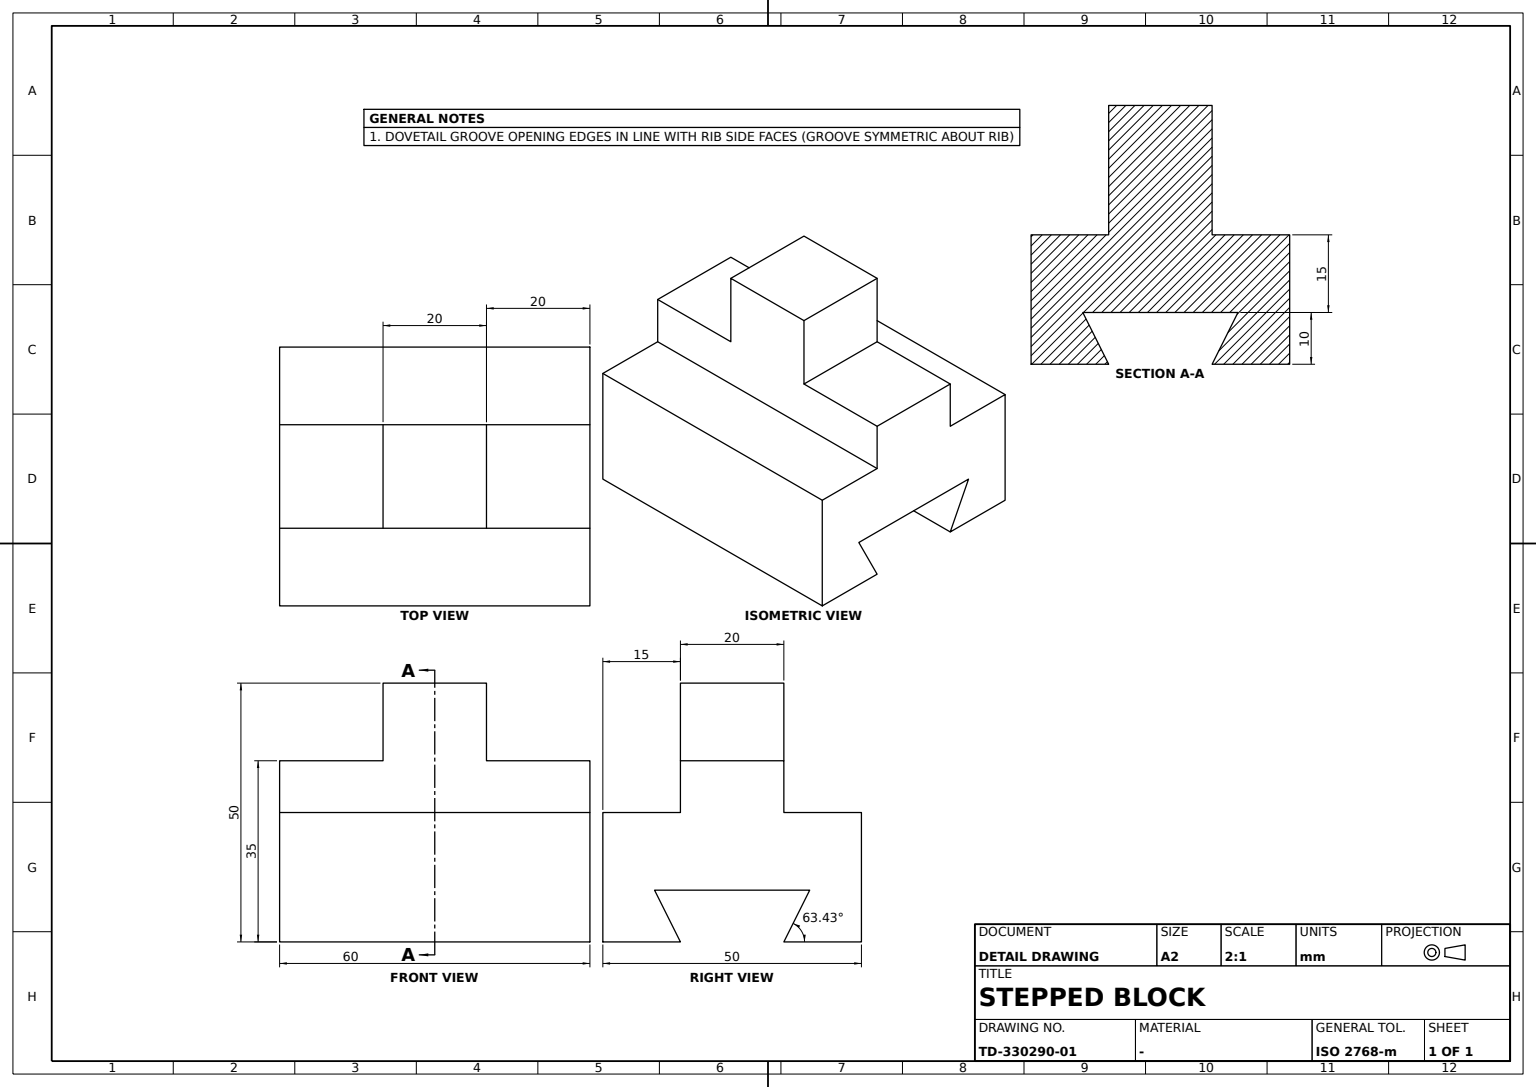
ISO-10303-21;
HEADER;
FILE_DESCRIPTION((''),'2;1');
FILE_NAME('','',(''),(''),'','','');
FILE_SCHEMA(('AUTOMOTIVE_DESIGN'));
ENDSEC;
DATA;
#1=APPLICATION_CONTEXT('');
#2=PRODUCT_CONTEXT('',#1,'mechanical');
#3=PRODUCT('','','',(#2));
#4=PRODUCT_DEFINITION_FORMATION('','',#3);
#5=PRODUCT_DEFINITION_CONTEXT('',#1,'design');
#6=PRODUCT_DEFINITION('','',#4,#5);
#7=PRODUCT_DEFINITION_SHAPE('','',#6);
#8=(LENGTH_UNIT()NAMED_UNIT(*)SI_UNIT(.MILLI.,.METRE.));
#9=(NAMED_UNIT(*)PLANE_ANGLE_UNIT()SI_UNIT($,.RADIAN.));
#10=(NAMED_UNIT(*)SI_UNIT($,.STERADIAN.)SOLID_ANGLE_UNIT());
#11=UNCERTAINTY_MEASURE_WITH_UNIT(LENGTH_MEASURE(0.005),#8,'distance_accuracy_value','');
#12=(GEOMETRIC_REPRESENTATION_CONTEXT(3)GLOBAL_UNCERTAINTY_ASSIGNED_CONTEXT((#11))GLOBAL_UNIT_ASSIGNED_CONTEXT((#8,#9,#10))REPRESENTATION_CONTEXT('',''));
#13=CARTESIAN_POINT('',(30.,-10.,-12.5));
#14=VERTEX_POINT('',#13);
#15=CARTESIAN_POINT('',(-30.,-10.,-12.5));
#16=VERTEX_POINT('',#15);
#17=CARTESIAN_POINT('',(60.,-10.,-12.5));
#18=DIRECTION('',(-1.,0.,0.));
#19=VECTOR('',#18,1000.);
#20=LINE('',#17,#19);
#21=EDGE_CURVE('',#14,#16,#20,.T.);
#22=ORIENTED_EDGE('',*,*,#21,.T.);
#23=CARTESIAN_POINT('',(-30.,-15.,-2.5));
#24=VERTEX_POINT('',#23);
#25=CARTESIAN_POINT('',(-30.,-13.,-6.5));
#26=DIRECTION('',(0.,-0.447213595,0.894427191));
#27=VECTOR('',#26,1000.);
#28=LINE('',#25,#27);
#29=EDGE_CURVE('',#16,#24,#28,.T.);
#30=ORIENTED_EDGE('',*,*,#29,.T.);
#31=CARTESIAN_POINT('',(30.,-15.,-2.5));
#32=VERTEX_POINT('',#31);
#33=CARTESIAN_POINT('',(60.,-15.,-2.5));
#34=LINE('',#33,#19);
#35=EDGE_CURVE('',#24,#32,#34,.F.);
#36=ORIENTED_EDGE('',*,*,#35,.T.);
#37=CARTESIAN_POINT('',(30.,-13.,-6.5));
#38=LINE('',#37,#27);
#39=EDGE_CURVE('',#14,#32,#38,.T.);
#40=ORIENTED_EDGE('',*,*,#39,.F.);
#41=EDGE_LOOP('',(#22,#30,#36,#40));
#42=FACE_BOUND('',#41,.T.);
#43=DIRECTION('',(0.,0.894427191,0.447213595));
#44=AXIS2_PLACEMENT_3D('',#33,#43,#26);
#45=PLANE('',#44);
#46=ADVANCED_FACE('',(#42),#45,.T.);
#47=CARTESIAN_POINT('',(10.,-10.,22.5));
#48=VERTEX_POINT('',#47);
#49=CARTESIAN_POINT('',(10.,-10.,37.5));
#50=VERTEX_POINT('',#49);
#51=DIRECTION('',(0.,0.,1.));
#52=VECTOR('',#51,1000.);
#53=LINE('',#47,#52);
#54=EDGE_CURVE('',#48,#50,#53,.T.);
#55=ORIENTED_EDGE('',*,*,#54,.F.);
#56=CARTESIAN_POINT('',(10.,10.,22.5));
#57=VERTEX_POINT('',#56);
#58=DIRECTION('',(0.,1.,0.));
#59=VECTOR('',#58,1000.);
#60=LINE('',#47,#59);
#61=EDGE_CURVE('',#48,#57,#60,.T.);
#62=ORIENTED_EDGE('',*,*,#61,.T.);
#63=CARTESIAN_POINT('',(10.,10.,37.5));
#64=VERTEX_POINT('',#63);
#65=LINE('',#56,#52);
#66=EDGE_CURVE('',#57,#64,#65,.T.);
#67=ORIENTED_EDGE('',*,*,#66,.T.);
#68=LINE('',#49,#59);
#69=EDGE_CURVE('',#50,#64,#68,.T.);
#70=ORIENTED_EDGE('',*,*,#69,.F.);
#71=EDGE_LOOP('',(#55,#62,#67,#70));
#72=FACE_BOUND('',#71,.T.);
#73=AXIS2_PLACEMENT_3D('',#47,#18,#51);
#74=PLANE('',#73);
#75=ADVANCED_FACE('',(#72),#74,.F.);
#76=CARTESIAN_POINT('',(-30.,-25.,12.5));
#77=VERTEX_POINT('',#76);
#78=CARTESIAN_POINT('',(-30.,-25.,-12.5));
#79=VERTEX_POINT('',#78);
#80=DIRECTION('',(0.,0.,-1.));
#81=VECTOR('',#80,1000.);
#82=LINE('',#76,#81);
#83=EDGE_CURVE('',#77,#79,#82,.T.);
#84=ORIENTED_EDGE('',*,*,#83,.F.);
#85=CARTESIAN_POINT('',(-30.,-10.,12.5));
#86=VERTEX_POINT('',#85);
#87=CARTESIAN_POINT('',(-30.,25.,12.5));
#88=DIRECTION('',(0.,-1.,0.));
#89=VECTOR('',#88,1000.);
#90=LINE('',#87,#89);
#91=EDGE_CURVE('',#86,#77,#90,.T.);
#92=ORIENTED_EDGE('',*,*,#91,.F.);
#93=CARTESIAN_POINT('',(-30.,-10.,22.5));
#94=VERTEX_POINT('',#93);
#95=LINE('',#85,#52);
#96=EDGE_CURVE('',#86,#94,#95,.T.);
#97=ORIENTED_EDGE('',*,*,#96,.T.);
#98=CARTESIAN_POINT('',(-30.,10.,22.5));
#99=VERTEX_POINT('',#98);
#100=LINE('',#93,#59);
#101=EDGE_CURVE('',#94,#99,#100,.T.);
#102=ORIENTED_EDGE('',*,*,#101,.T.);
#103=CARTESIAN_POINT('',(-30.,10.,12.5));
#104=VERTEX_POINT('',#103);
#105=LINE('',#98,#81);
#106=EDGE_CURVE('',#99,#104,#105,.T.);
#107=ORIENTED_EDGE('',*,*,#106,.T.);
#108=VERTEX_POINT('',#87);
#109=EDGE_CURVE('',#108,#104,#90,.T.);
#110=ORIENTED_EDGE('',*,*,#109,.F.);
#111=CARTESIAN_POINT('',(-30.,25.,-12.5));
#112=VERTEX_POINT('',#111);
#113=LINE('',#111,#52);
#114=EDGE_CURVE('',#112,#108,#113,.T.);
#115=ORIENTED_EDGE('',*,*,#114,.F.);
#116=CARTESIAN_POINT('',(-30.,10.,-12.5));
#117=VERTEX_POINT('',#116);
#118=LINE('',#78,#59);
#119=EDGE_CURVE('',#117,#112,#118,.T.);
#120=ORIENTED_EDGE('',*,*,#119,.F.);
#121=CARTESIAN_POINT('',(-30.,15.,-2.5));
#122=VERTEX_POINT('',#121);
#123=CARTESIAN_POINT('',(-30.,13.,-6.5));
#124=DIRECTION('',(0.,-0.447213595,-0.894427191));
#125=VECTOR('',#124,1000.);
#126=LINE('',#123,#125);
#127=EDGE_CURVE('',#122,#117,#126,.T.);
#128=ORIENTED_EDGE('',*,*,#127,.F.);
#129=CARTESIAN_POINT('',(-30.,0.,-2.5));
#130=LINE('',#129,#59);
#131=EDGE_CURVE('',#24,#122,#130,.T.);
#132=ORIENTED_EDGE('',*,*,#131,.F.);
#133=ORIENTED_EDGE('',*,*,#29,.F.);
#134=EDGE_CURVE('',#79,#16,#118,.T.);
#135=ORIENTED_EDGE('',*,*,#134,.F.);
#136=EDGE_LOOP('',(#84,#92,#97,#102,#107,#110,#115,#120,#128,#132,#133,#135));
#137=FACE_BOUND('',#136,.T.);
#138=CARTESIAN_POINT('',(-30.,0.,0.));
#139=DIRECTION('',(1.,0.,0.));
#140=AXIS2_PLACEMENT_3D('',#138,#139,#80);
#141=PLANE('',#140);
#142=ADVANCED_FACE('',(#137),#141,.F.);
#143=CARTESIAN_POINT('',(30.,25.,-12.5));
#144=VERTEX_POINT('',#143);
#145=CARTESIAN_POINT('',(30.,25.,12.5));
#146=VERTEX_POINT('',#145);
#147=LINE('',#143,#52);
#148=EDGE_CURVE('',#144,#146,#147,.T.);
#149=ORIENTED_EDGE('',*,*,#148,.F.);
#150=LINE('',#143,#19);
#151=EDGE_CURVE('',#144,#112,#150,.T.);
#152=ORIENTED_EDGE('',*,*,#151,.T.);
#153=ORIENTED_EDGE('',*,*,#114,.T.);
#154=LINE('',#145,#19);
#155=EDGE_CURVE('',#146,#108,#154,.T.);
#156=ORIENTED_EDGE('',*,*,#155,.F.);
#157=EDGE_LOOP('',(#149,#152,#153,#156));
#158=FACE_BOUND('',#157,.T.);
#159=AXIS2_PLACEMENT_3D('',#143,#88,#80);
#160=PLANE('',#159);
#161=ADVANCED_FACE('',(#158),#160,.F.);
#162=CARTESIAN_POINT('',(30.,-25.,-12.5));
#163=VERTEX_POINT('',#162);
#164=LINE('',#162,#19);
#165=EDGE_CURVE('',#163,#79,#164,.T.);
#166=ORIENTED_EDGE('',*,*,#165,.F.);
#167=CARTESIAN_POINT('',(30.,-25.,12.5));
#168=VERTEX_POINT('',#167);
#169=LINE('',#167,#81);
#170=EDGE_CURVE('',#168,#163,#169,.T.);
#171=ORIENTED_EDGE('',*,*,#170,.F.);
#172=LINE('',#167,#19);
#173=EDGE_CURVE('',#168,#77,#172,.T.);
#174=ORIENTED_EDGE('',*,*,#173,.T.);
#175=ORIENTED_EDGE('',*,*,#83,.T.);
#176=EDGE_LOOP('',(#166,#171,#174,#175));
#177=FACE_BOUND('',#176,.T.);
#178=AXIS2_PLACEMENT_3D('',#167,#58,#51);
#179=PLANE('',#178);
#180=ADVANCED_FACE('',(#177),#179,.F.);
#181=ORIENTED_EDGE('',*,*,#96,.F.);
#182=CARTESIAN_POINT('',(30.,-10.,12.5));
#183=VERTEX_POINT('',#182);
#184=LINE('',#182,#19);
#185=EDGE_CURVE('',#183,#86,#184,.T.);
#186=ORIENTED_EDGE('',*,*,#185,.F.);
#187=CARTESIAN_POINT('',(30.,-10.,22.5));
#188=VERTEX_POINT('',#187);
#189=LINE('',#182,#52);
#190=EDGE_CURVE('',#183,#188,#189,.T.);
#191=ORIENTED_EDGE('',*,*,#190,.T.);
#192=LINE('',#187,#19);
#193=EDGE_CURVE('',#188,#48,#192,.T.);
#194=ORIENTED_EDGE('',*,*,#193,.T.);
#195=ORIENTED_EDGE('',*,*,#54,.T.);
#196=CARTESIAN_POINT('',(-10.,-10.,37.5));
#197=VERTEX_POINT('',#196);
#198=LINE('',#49,#19);
#199=EDGE_CURVE('',#50,#197,#198,.T.);
#200=ORIENTED_EDGE('',*,*,#199,.T.);
#201=CARTESIAN_POINT('',(-10.,-10.,22.5));
#202=VERTEX_POINT('',#201);
#203=LINE('',#196,#81);
#204=EDGE_CURVE('',#197,#202,#203,.T.);
#205=ORIENTED_EDGE('',*,*,#204,.T.);
#206=EDGE_CURVE('',#202,#94,#192,.T.);
#207=ORIENTED_EDGE('',*,*,#206,.T.);
#208=EDGE_LOOP('',(#181,#186,#191,#194,#195,#200,#205,#207));
#209=FACE_BOUND('',#208,.T.);
#210=AXIS2_PLACEMENT_3D('',#182,#88,#80);
#211=PLANE('',#210);
#212=ADVANCED_FACE('',(#209),#211,.T.);
#213=CARTESIAN_POINT('',(30.,10.,12.5));
#214=VERTEX_POINT('',#213);
#215=LINE('',#213,#19);
#216=EDGE_CURVE('',#214,#104,#215,.T.);
#217=ORIENTED_EDGE('',*,*,#216,.T.);
#218=ORIENTED_EDGE('',*,*,#106,.F.);
#219=CARTESIAN_POINT('',(-10.,10.,22.5));
#220=VERTEX_POINT('',#219);
#221=CARTESIAN_POINT('',(30.,10.,22.5));
#222=LINE('',#221,#19);
#223=EDGE_CURVE('',#220,#99,#222,.T.);
#224=ORIENTED_EDGE('',*,*,#223,.F.);
#225=CARTESIAN_POINT('',(-10.,10.,37.5));
#226=VERTEX_POINT('',#225);
#227=LINE('',#225,#81);
#228=EDGE_CURVE('',#226,#220,#227,.T.);
#229=ORIENTED_EDGE('',*,*,#228,.F.);
#230=LINE('',#63,#19);
#231=EDGE_CURVE('',#64,#226,#230,.T.);
#232=ORIENTED_EDGE('',*,*,#231,.F.);
#233=ORIENTED_EDGE('',*,*,#66,.F.);
#234=VERTEX_POINT('',#221);
#235=EDGE_CURVE('',#234,#57,#222,.T.);
#236=ORIENTED_EDGE('',*,*,#235,.F.);
#237=LINE('',#221,#81);
#238=EDGE_CURVE('',#234,#214,#237,.T.);
#239=ORIENTED_EDGE('',*,*,#238,.T.);
#240=EDGE_LOOP('',(#217,#218,#224,#229,#232,#233,#236,#239));
#241=FACE_BOUND('',#240,.T.);
#242=AXIS2_PLACEMENT_3D('',#221,#58,#51);
#243=PLANE('',#242);
#244=ADVANCED_FACE('',(#241),#243,.T.);
#245=ORIENTED_EDGE('',*,*,#228,.T.);
#246=LINE('',#201,#59);
#247=EDGE_CURVE('',#202,#220,#246,.T.);
#248=ORIENTED_EDGE('',*,*,#247,.F.);
#249=ORIENTED_EDGE('',*,*,#204,.F.);
#250=LINE('',#196,#59);
#251=EDGE_CURVE('',#197,#226,#250,.T.);
#252=ORIENTED_EDGE('',*,*,#251,.T.);
#253=EDGE_LOOP('',(#245,#248,#249,#252));
#254=FACE_BOUND('',#253,.T.);
#255=AXIS2_PLACEMENT_3D('',#196,#139,#80);
#256=PLANE('',#255);
#257=ADVANCED_FACE('',(#254),#256,.F.);
#258=LINE('',#145,#89);
#259=EDGE_CURVE('',#183,#168,#258,.T.);
#260=ORIENTED_EDGE('',*,*,#259,.F.);
#261=ORIENTED_EDGE('',*,*,#185,.T.);
#262=ORIENTED_EDGE('',*,*,#91,.T.);
#263=ORIENTED_EDGE('',*,*,#173,.F.);
#264=EDGE_LOOP('',(#260,#261,#262,#263));
#265=FACE_BOUND('',#264,.T.);
#266=AXIS2_PLACEMENT_3D('',#145,#80,#18);
#267=PLANE('',#266);
#268=ADVANCED_FACE('',(#265),#267,.F.);
#269=ORIENTED_EDGE('',*,*,#223,.T.);
#270=ORIENTED_EDGE('',*,*,#101,.F.);
#271=ORIENTED_EDGE('',*,*,#206,.F.);
#272=ORIENTED_EDGE('',*,*,#247,.T.);
#273=EDGE_LOOP('',(#269,#270,#271,#272));
#274=FACE_BOUND('',#273,.T.);
#275=AXIS2_PLACEMENT_3D('',#187,#51,#139);
#276=PLANE('',#275);
#277=ADVANCED_FACE('',(#274),#276,.T.);
#278=ORIENTED_EDGE('',*,*,#193,.F.);
#279=LINE('',#187,#59);
#280=EDGE_CURVE('',#188,#234,#279,.T.);
#281=ORIENTED_EDGE('',*,*,#280,.T.);
#282=ORIENTED_EDGE('',*,*,#235,.T.);
#283=ORIENTED_EDGE('',*,*,#61,.F.);
#284=EDGE_LOOP('',(#278,#281,#282,#283));
#285=FACE_BOUND('',#284,.T.);
#286=ADVANCED_FACE('',(#285),#276,.T.);
#287=ORIENTED_EDGE('',*,*,#69,.T.);
#288=ORIENTED_EDGE('',*,*,#231,.T.);
#289=ORIENTED_EDGE('',*,*,#251,.F.);
#290=ORIENTED_EDGE('',*,*,#199,.F.);
#291=EDGE_LOOP('',(#287,#288,#289,#290));
#292=FACE_BOUND('',#291,.T.);
#293=AXIS2_PLACEMENT_3D('',#49,#80,#18);
#294=PLANE('',#293);
#295=ADVANCED_FACE('',(#292),#294,.F.);
#296=ORIENTED_EDGE('',*,*,#119,.T.);
#297=ORIENTED_EDGE('',*,*,#151,.F.);
#298=CARTESIAN_POINT('',(30.,10.,-12.5));
#299=VERTEX_POINT('',#298);
#300=LINE('',#162,#59);
#301=EDGE_CURVE('',#299,#144,#300,.T.);
#302=ORIENTED_EDGE('',*,*,#301,.F.);
#303=CARTESIAN_POINT('',(60.,10.,-12.5));
#304=LINE('',#303,#19);
#305=EDGE_CURVE('',#299,#117,#304,.T.);
#306=ORIENTED_EDGE('',*,*,#305,.T.);
#307=EDGE_LOOP('',(#296,#297,#302,#306));
#308=FACE_BOUND('',#307,.T.);
#309=AXIS2_PLACEMENT_3D('',#162,#51,#139);
#310=PLANE('',#309);
#311=ADVANCED_FACE('',(#308),#310,.F.);
#312=ORIENTED_EDGE('',*,*,#35,.F.);
#313=ORIENTED_EDGE('',*,*,#131,.T.);
#314=CARTESIAN_POINT('',(30.,15.,-2.5));
#315=VERTEX_POINT('',#314);
#316=CARTESIAN_POINT('',(60.,15.,-2.5));
#317=LINE('',#316,#19);
#318=EDGE_CURVE('',#122,#315,#317,.F.);
#319=ORIENTED_EDGE('',*,*,#318,.T.);
#320=CARTESIAN_POINT('',(30.,0.,-2.5));
#321=LINE('',#320,#59);
#322=EDGE_CURVE('',#32,#315,#321,.T.);
#323=ORIENTED_EDGE('',*,*,#322,.F.);
#324=EDGE_LOOP('',(#312,#313,#319,#323));
#325=FACE_BOUND('',#324,.T.);
#326=AXIS2_PLACEMENT_3D('',#316,#80,#18);
#327=PLANE('',#326);
#328=ADVANCED_FACE('',(#325),#327,.T.);
#329=ORIENTED_EDGE('',*,*,#190,.F.);
#330=ORIENTED_EDGE('',*,*,#259,.T.);
#331=ORIENTED_EDGE('',*,*,#170,.T.);
#332=EDGE_CURVE('',#163,#14,#300,.T.);
#333=ORIENTED_EDGE('',*,*,#332,.T.);
#334=ORIENTED_EDGE('',*,*,#39,.T.);
#335=ORIENTED_EDGE('',*,*,#322,.T.);
#336=CARTESIAN_POINT('',(30.,13.,-6.5));
#337=LINE('',#336,#125);
#338=EDGE_CURVE('',#315,#299,#337,.T.);
#339=ORIENTED_EDGE('',*,*,#338,.T.);
#340=ORIENTED_EDGE('',*,*,#301,.T.);
#341=ORIENTED_EDGE('',*,*,#148,.T.);
#342=EDGE_CURVE('',#146,#214,#258,.T.);
#343=ORIENTED_EDGE('',*,*,#342,.T.);
#344=ORIENTED_EDGE('',*,*,#238,.F.);
#345=ORIENTED_EDGE('',*,*,#280,.F.);
#346=EDGE_LOOP('',(#329,#330,#331,#333,#334,#335,#339,#340,#341,#343,#344,#345));
#347=FACE_BOUND('',#346,.T.);
#348=CARTESIAN_POINT('',(30.,0.,0.));
#349=AXIS2_PLACEMENT_3D('',#348,#139,#80);
#350=PLANE('',#349);
#351=ADVANCED_FACE('',(#347),#350,.T.);
#352=ORIENTED_EDGE('',*,*,#21,.F.);
#353=ORIENTED_EDGE('',*,*,#332,.F.);
#354=ORIENTED_EDGE('',*,*,#165,.T.);
#355=ORIENTED_EDGE('',*,*,#134,.T.);
#356=EDGE_LOOP('',(#352,#353,#354,#355));
#357=FACE_BOUND('',#356,.T.);
#358=ADVANCED_FACE('',(#357),#310,.F.);
#359=ORIENTED_EDGE('',*,*,#338,.F.);
#360=ORIENTED_EDGE('',*,*,#318,.F.);
#361=ORIENTED_EDGE('',*,*,#127,.T.);
#362=ORIENTED_EDGE('',*,*,#305,.F.);
#363=EDGE_LOOP('',(#359,#360,#361,#362));
#364=FACE_BOUND('',#363,.T.);
#365=DIRECTION('',(0.,-0.894427191,0.447213595));
#366=AXIS2_PLACEMENT_3D('',#303,#365,#124);
#367=PLANE('',#366);
#368=ADVANCED_FACE('',(#364),#367,.T.);
#369=ORIENTED_EDGE('',*,*,#342,.F.);
#370=ORIENTED_EDGE('',*,*,#155,.T.);
#371=ORIENTED_EDGE('',*,*,#109,.T.);
#372=ORIENTED_EDGE('',*,*,#216,.F.);
#373=EDGE_LOOP('',(#369,#370,#371,#372));
#374=FACE_BOUND('',#373,.T.);
#375=ADVANCED_FACE('',(#374),#267,.F.);
#376=CLOSED_SHELL('',(#46,#75,#142,#161,#180,#212,#244,#257,#268,#277,#286,#295,#311,#328,#351,#358,#368,#375));
#377=MANIFOLD_SOLID_BREP('',#376);
#378=ADVANCED_BREP_SHAPE_REPRESENTATION('',(#377),#12);
#379=SHAPE_DEFINITION_REPRESENTATION(#7,#378);
ENDSEC;
END-ISO-10303-21;
